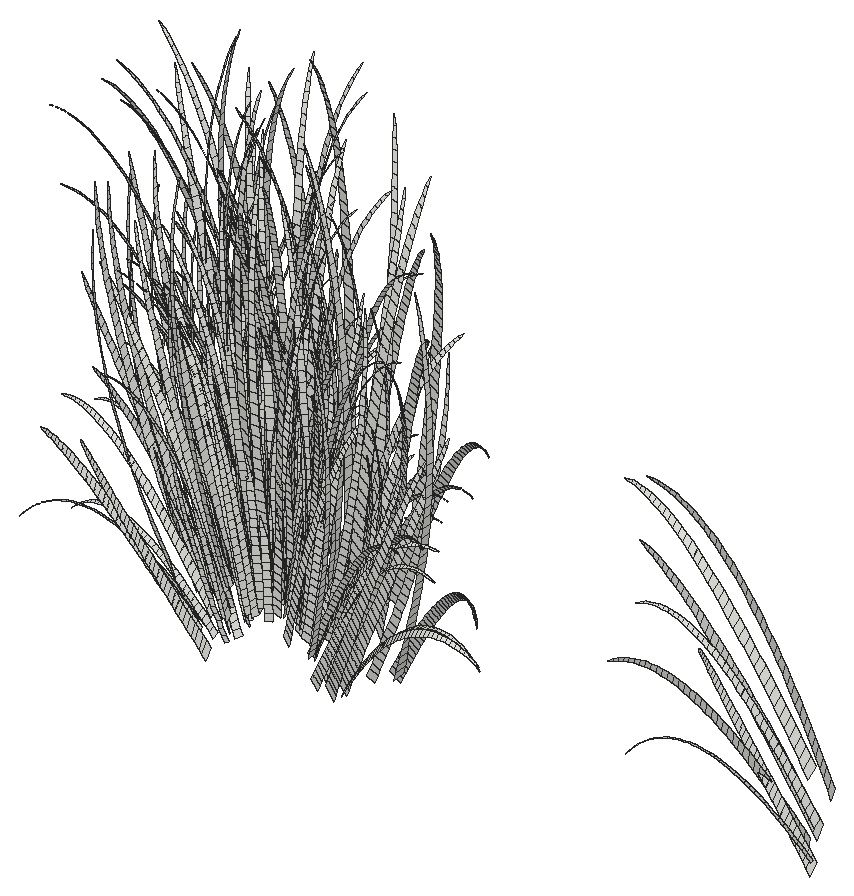
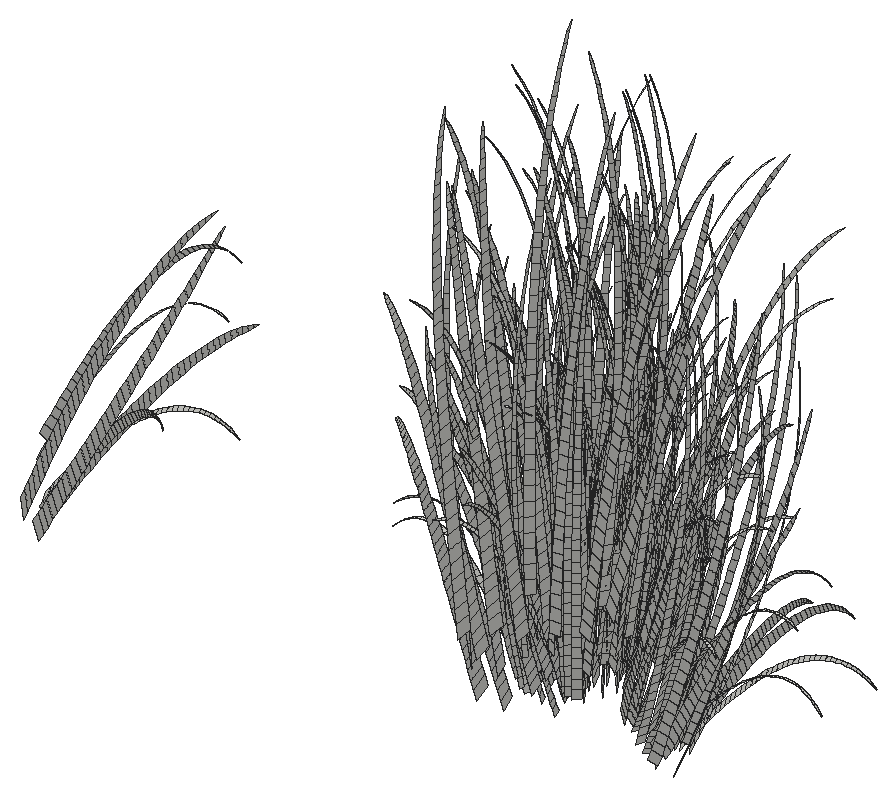
# SketchUp Ruby script. Lengths in inches.
U = 1.inch
M = Sketchup.active_model
def pt(a) = Geom::Point3d.new(a.map { |v| v * U })
def face(e, loops, mat)
  f = e.add_face(loops[0].map { |a| pt(a) })
  loops[1..].each { |l| e.add_face(l.map { |a| pt(a) }).erase! }
  f.material = f.back_material = mat if mat
  f
end
# faces: each face lists its corners as indices into pts; further lists are holes
def faces(e, pts, list, mat = nil) = list.each { |f| face(e, (f[0].is_a?(Array) ? f : [f]).map { |l| l.map { |i| pts[i] } }, mat) }
# xy, xz, yz: faces in a plane at the given z, y or x. An outline is a flat list of corners, or four numbers for a rectangle; further outlines are holes
def ring(l) = l.size == 4 ? [[l[0], l[1]], [l[2], l[1]], [l[2], l[3]], [l[0], l[3]]] : l.each_slice(2).to_a
def flat(e, list, mat, &to3) = list.each { |f| face(e, (f[0].is_a?(Array) ? f : [f]).map { |l| ring(l).map { |u, v| to3.(u, v) } }, mat) }
def xy(e, z, list, mat = nil) = flat(e, list, mat) { |x, y| [x, y, z] }
def xz(e, y, list, mat = nil) = flat(e, list, mat) { |x, z| [x, y, z] }
def yz(e, x, list, mat = nil) = flat(e, list, mat) { |y, z| [x, y, z] }
def lines(e, pts, list) = list.each { |a, b| e.add_line(pt(pts[a]), pt(pts[b])) }
# prism: a flat outline (further loops are holes) pulled along v
def prism(e, loops, v, mat = nil)
  f = face(e, loops, mat); d = Geom::Vector3d.new(v.map { |x| x * U })
  f.pushpull(f.normal.samedirection?(d) ? d.length : -d.length)
end
def box(e, o, s, mat = nil) = prism(e, [[o, [o[0] + s[0], o[1], o[2]], [o[0] + s[0], o[1] + s[1], o[2]], [o[0], o[1] + s[1], o[2]]]], [0, 0, s[2]], mat)
def at(x, y, z, deg = 0) = Geom::Transformation.translation(pt([x, y, z])) * Geom::Transformation.rotation(ORIGIN, Z_AXIS, deg.degrees)
def axes(o, x, y, z) = Geom::Transformation.new([*x, 0, *y, 0, *z, 0, *pt(o).to_a, 1])
def part(name) = M.definitions.add(name)
# library, detail: a bought-in or finely detailed component or shape, given as its bounding box
def library(name, o, s) = part(name).tap { |d| box(d.entities, o, s) }
def detail(e, o, s) = box(e.add_group.entities, o, s)
def put(e, d, t, mat = nil) = e.add_instance(d, t).tap { |i| i.material = mat if mat }
def group(e, t, mat = nil) = e.add_group.tap { |g| g.transformation = t; g.material = mat if mat }.entities
root = M.entities
c1 = part("fur_instance\#8")
p = [[-0.25,1.49,0.03],[0.25,-1.49,-0.03],[0.44,-1.47,1.51],[-0.05,1.47,1.57],[0.65,-1.44,3.05],[0.16,1.45,3.11],
  [0.86,-1.42,4.59],[0.38,1.44,4.65],[1.1,-1.39,6.13],[0.62,1.43,6.18],[1.34,-1.35,7.66],[0.875,1.42,7.72],
  [1.6,-1.32,9.19],[1.14,1.41,9.25],[1.88,-1.28,10.72],[1.43,1.41,10.78],[2.18,-1.24,12.25],[1.73,1.41,12.3],
  [2.49,-1.19,13.77],[2.05,1.41,13.82],[2.83,-1.15,15.29],[2.4,1.41,15.34],[3.18,-1.09,16.8],[2.76,1.42,16.85],
  [3.56,-1.03,18.31],[3.14,1.43,18.35],[3.96,-0.97,19.81],[3.55,1.44,19.85],[4.38,-0.91,21.3],[3.99,1.46,21.35],
  [4.84,-0.83,22.78],[4.45,1.48,22.83],[5.32,-0.76,24.26],[4.93,1.51,24.31],[5.82,-0.67,25.73],[5.45,1.54,25.77],
  [6.36,-0.59,27.18],[6,1.57,27.23],[6.93,-0.49,28.625],[6.58,1.61,28.67],[7.54,-0.39,30.05],[7.19,1.66,30.1],
  [8.18,-0.28,31.47],[7.84,1.71,31.51],[8.85,-0.16,32.86],[8.53,1.77,32.9],[9.57,-0.04,34.24],[9.25,1.83,34.27],
  [10.32,0.09,35.59],[10.02,1.9,35.625],[11.12,0.23,36.92],[10.82,1.97,36.95],[11.95,0.38,38.22],[11.67,2.06,38.25],
  [12.84,0.54,39.49],[12.57,2.14,39.52],[13.76,0.71,40.73],[13.51,2.24,40.76],[14.73,0.89,41.93],[14.49,2.34,41.95],
  [15.75,1.08,43.09],[15.52,2.45,43.11],[16.82,1.28,44.2],[16.6,2.5625,44.23],[17.93,1.5,45.27],[17.73,2.68,45.29],
  [19.08,1.73,46.28],[18.9,2.81,46.3],[20.29,1.97,47.24],[20.125,2.93,47.26],[21.53,2.22,48.13],[21.39,3.0625,48.15],
  [22.82,2.5,48.96],[22.7,3.1875,48.98],[24.14,2.8125,49.72],[24.06,3.3,49.73],[25.48,3.27,50.41]]
faces(c1.entities,p,[[0,1,2,3],[3,2,4,5],[5,4,6,7],[7,6,8,9],[9,8,10,11],[11,10,12,13],[13,12,14,15],[15,14,16,17],
  [17,16,18,19],[19,18,20,21],[21,20,22,23],[23,22,24,25],[25,24,26,27],[27,26,28,29],[29,28,30,31],[31,30,32,33],
  [33,32,34,35],[35,34,36,37],[37,36,38,39],[39,38,40,41],[41,40,42,43],[43,42,44,45],[45,44,46,47],[47,46,48,49],
  [49,48,50,51],[51,50,52,53],[53,52,54,55],[55,54,56,57],[57,56,58,59],[59,58,60,61],[61,60,62,63],[63,62,64,65],
  [65,64,66,67],[67,66,68,69],[69,68,70,71],[71,70,72,73],[73,72,74,75],[75,74,76]])
put(root,c1,axes([160.64,67.0625,2.47],[-0.11039,-0.00414,-0.3495],[0.07669,-0.1786,0.00651],[-0.14786,-0.06719,0.2791]))
put(root,c1,axes([161.22,65.8125,2.49],[-0.13594,0.15084,-0.11164],[-0.0609,-0.07291,-0.33491],[-0.13519,-0.09407,0.27953]))
put(root,c1,axes([158.93,69.58,2.69],[0.13391,-0.00422,0.37894],[-0.02725,0.21287,-0.08205],[-0.17659,-0.01268,0.31548]))
put(root,c1,axes([161.61,66.53,3.77],[-0.14992,0.10635,-0.20855],[-0.03569,-0.13875,-0.18978],[-0.12006,-0.06524,0.33426]))
put(root,c1,axes([161.6,67.96,3.64],[-0.13947,0.07457,-0.26376],[-0.03048,-0.16347,-0.05841],[-0.12421,-0.01975,0.3263]))
put(root,c1,axes([161.64,66.7,2.23],[-0.11214,0.07357,-0.29467],[-0.00419,-0.1506,-0.10442],[-0.13991,-0.03543,0.25192]))
put(root,c1,axes([160.7,70.26,10.22],[-0.16722,-0.14584,-0.14657],[0.18274,-0.19209,0.09427],[-0.0816,-0.06233,0.55718]))
put(root,c1,axes([159.23,71.21,3.75],[0.10956,-0.18152,0.25882],[0.13509,0.11782,0.19082],[-0.14519,0.00192,0.39222]))
put(root,c1,axes([160.22,69.17,3.12],[0.07012,-0.18381,0.20265],[0.10518,0.07075,0.29594],[-0.16336,-0.01173,0.29184]))
put(root,c1,axes([160.11,66.95,2.47],[0.11177,0.01694,0.37048],[-0.08915,0.18926,-0.03147],[-0.15727,-0.07147,0.29687]))
put(root,c1,axes([160.63,67.58,2.98],[0.07273,0.09595,0.27862],[-0.10249,0.16133,-0.212],[-0.15668,-0.03967,0.28211]))
put(root,c1,axes([159.15,68.47,3.74],[0.16226,-0.13696,0.26442],[0.06401,0.16282,0.19515],[-0.14822,-0.05035,0.39313]))
put(root,c1,axes([161.99,68.57,8.76],[-0.19486,-0.07064,-0.15993],[0.11436,-0.20339,0.01183],[-0.07048,-0.06892,0.50496]))
put(root,c1,axes([162.2,65.35,1.82],[-0.09839,0.14314,-0.01192],[-0.08354,-0.02419,-0.30566],[-0.11714,-0.08151,0.24221]))
put(root,c1,axes([161.59,68.2,2.32],[-0.01321,-0.17005,0.06481],[0.1141,-0.02557,0.30569],[-0.13946,0.01456,0.25678]))
put(root,c1,axes([162.7,69.16,6.58],[-0.18243,0.01895,-0.19563],[-0.00133,-0.1948,0.08688],[-0.09334,0.00298,0.40574]))
put(root,c1,axes([162.57,67.88,4.63],[-0.16023,0.03354,-0.19126],[-0.00898,-0.17162,0.02853],[-0.08895,-0.01176,0.36236]))
put(root,c1,axes([162.53,66.625,5.96],[-0.1494,0.14445,-0.05993],[-0.10862,-0.10225,-0.21391],[-0.08642,-0.08137,0.39881]))
put(root,c1,axes([160.01,68.125,4.63],[0.16036,-0.12824,0.26431],[0.05712,0.1633,0.18167],[-0.14465,-0.04914,0.38366]))
put(root,c1,axes([160.43,68.18,3.85],[0.12489,0.06673,0.27563],[-0.09958,0.18305,-0.12082],[-0.13573,-0.04611,0.36]))
put(root,c1,axes([162.82,66.73,4.46],[-0.15052,-0.00251,-0.18515],[0.03159,-0.16716,0.03488],[-0.08794,-0.02622,0.34898]))
put(root,c1,axes([162.91,68.06,3.03],[-0.10384,0.1021,-0.23208],[-0.0841,-0.12138,-0.04288],[-0.10059,0.0191,0.29067]))
put(root,c1,axes([162.55,68.69,5.18],[-0.10618,-0.13262,-0.04878],[0.13367,-0.1263,0.19427],[-0.08735,0.00279,0.37967]))
put(root,c1,axes([161.4,68.18,1.81],[0.10833,0.05099,0.24664],[-0.03776,0.16401,-0.19126],[-0.1393,0.01454,0.25647]))
put(root,c1,axes([162.52,70.78,11.4],[-0.09372,-0.20637,-0.07363],[0.22677,-0.12712,0.15354],[-0.08199,-0.04812,0.55353]))
put(root,c1,axes([160.94,69.19,4.28],[0.15491,-0.05585,0.29054],[0.02871,0.18789,-0.02061],[-0.13151,0.00174,0.35528]))
put(root,c1,axes([163.55,67.92,5.72],[-0.13836,0.10656,-0.19014],[-0.08729,-0.13946,-0.02631],[-0.08371,0.00267,0.36384]))
put(root,c1,axes([162.43,66.87,3.52],[0.03066,0.14936,0.05869],[-0.12804,0.07175,-0.24213],[-0.11455,-0.01821,0.30092]))
put(root,c1,axes([162.8,66.9375,7.41],[-0.03053,0.18634,0.11663],[-0.19498,0.03215,-0.20672],[-0.09234,-0.08694,0.42611]))
put(root,c1,axes([163.05,66.09,6],[-0.076,0.1669,0.09562],[-0.17144,-0.01335,-0.19918],[-0.07397,-0.09509,0.39348]))
put(root,c1,axes([163.36,67.9,6.33],[-0.14595,-0.08896,-0.08701],[0.11069,-0.159,0.08949],[-0.05969,-0.02587,0.41282]))
put(root,c1,axes([163.37,66.87,6.51],[-0.13003,0.1505,-0.04051],[-0.13515,-0.09639,-0.12681],[-0.0585,-0.05721,0.41915]))
put(root,c1,axes([163.36,69.73,10.31],[-0.20007,-0.1011,-0.05198],[0.13259,-0.20105,0.02025],[-0.03025,-0.05245,0.53866]))
put(root,c1,axes([163.86,69.61,11.42],[-0.23914,-0.05106,-0.06078],[0.08551,-0.22855,-0.0252],[-0.02809,-0.06875,0.5682]))
put(root,c1,axes([162.3,67.93,1.8125],[0.06974,-0.11239,0.27242],[0.09117,0.10684,0.0892],[-0.12045,0.03482,0.23783]))
put(root,c1,axes([161.48,69.49,3.4],[0.12819,-0.10555,0.27193],[0.08655,0.15023,0.02614],[-0.11644,0.02211,0.33646]))
put(root,c1,axes([162.47,66.64,2.11],[0.09888,-0.02928,0.28041],[-0.00291,0.15131,-0.01175],[-0.12783,-0.00918,0.22836]))
put(root,c1,axes([162.99,68.41,3.74],[-0.01787,-0.16163,0.13786],[0.14541,-0.01364,0.20157],[-0.09392,0.03632,0.30351]))
put(root,c1,axes([163.91,66.9,5.53],[-0.15295,0.08658,-0.10984],[-0.06653,-0.14152,-0.02919],[-0.05435,-0.02356,0.3759]))
put(root,c1,axes([163.57,68.36,3.76],[-0.08732,-0.12975,0.07004],[0.12156,-0.08169,0.22443],[-0.07712,0.04857,0.29461]))
put(root,c1,axes([164.39,69.47,11.48],[-0.24023,0.10194,-0.01182],[-0.08393,-0.20819,-0.06775],[-0.02132,-0.07588,0.56748]))
put(root,c1,axes([162.11,66.95,3.46],[0.13512,-0.04534,0.25565],[0.00767,0.16418,0.01521],[-0.11775,-0.01872,0.30933]))
put(root,c1,axes([164.27,66.88,5.49],[-0.16155,0.04363,-0.11105],[-0.02173,-0.15615,0.00187],[-0.05311,-0.02302,0.36735]))
put(root,c1,axes([164.18,68.14,5.39],[-0.13763,-0.08778,-0.02445],[0.09224,-0.14199,0.18002],[-0.06167,0.02548,0.35158]))
put(root,c1,axes([163.87,67.91,9.83],[-0.11071,0.19643,0.08485],[-0.20741,-0.05916,-0.14436],[-0.04649,-0.10158,0.50968]))
put(root,c1,axes([162.19,67.375,5.75],[0.12398,0.09622,0.18511],[-0.12468,0.16008,-0.11198],[-0.09878,-0.04719,0.39625]))
put(root,c1,axes([164.5,67.29,6.31],[-0.15275,-0.06369,-0.07605],[0.08272,-0.1606,0.08732],[-0.05298,-0.01559,0.38969]))
put(root,c1,axes([164.34,66.44,5.47],[-0.12167,0.12231,-0.08026],[-0.10576,-0.10199,-0.07795],[-0.05387,-0.03162,0.36369]))
put(root,c1,axes([162.84,67.73,5.89],[0.1073,0.11537,0.13468],[-0.12896,0.14123,-0.15523],[-0.09593,-0.0286,0.38067]))
put(root,c1,axes([164.74,66.98,5.32],[-0.15222,0.06371,-0.10078],[-0.04912,-0.14483,0.02613],[-0.04368,-0.00705,0.35627]))
put(root,c1,axes([164.89,66.57,7.14],[-0.18454,0.07316,-0.01839],[-0.05778,-0.16138,-0.04792],[-0.01906,-0.05522,0.43193]))
put(root,c1,axes([163.59,71.5625,10.07],[-0.03022,-0.22611,0.09029],[0.23429,-0.05028,0.11994],[-0.05481,-0.00145,0.5217]))
put(root,c1,axes([163.08,65.9,6.21],[0.08886,0.11953,0.22309],[-0.17307,0.12603,-0.0526],[-0.07674,-0.09865,0.40821]))
put(root,c1,axes([165,69.69,10.62],[-0.19122,-0.11806,-0.01455],[0.14538,-0.19433,0.04316],[-0.02276,-0.03764,0.53822]))
put(root,c1,axes([164,68.76,6.79],[-0.07059,-0.16734,0.04684],[0.17777,-0.08469,0.11217],[-0.04438,-0.00118,0.42241]))
put(root,c1,axes([165.09,67.4,6.18],[-0.1632,-0.04584,-0.02491],[0.06111,-0.16287,0.10545],[-0.03205,0.00396,0.38155]))
put(root,c1,axes([164.32,67.78,5.81],[-0.07809,-0.14325,0.0107],[0.15359,-0.09235,0.11164],[-0.04706,-0.00759,0.38378]))
put(root,c1,axes([165.17,68.24,7.07],[-0.18597,0.0618,-0.02273],[-0.04748,-0.17087,0.02426],[-0.01189,-0.02692,0.4292]))
put(root,c1,axes([163.43,67.35,3.28],[0.12505,0.02128,0.17693],[-0.02026,0.14885,-0.13694],[-0.09536,0.01811,0.27556]))
put(root,c1,axes([161.55,70.37,10.29],[0.23978,-0.07082,0.15768],[0.03022,0.22441,0.06362],[-0.07961,-0.06081,0.54364]))
put(root,c1,axes([164.3,68.31,8.43],[-0.04674,0.1979,-0.00041],[-0.20698,-0.02041,-0.04932],[-0.02674,-0.04637,0.47621]))
put(root,c1,axes([161.95,68.09,9.79],[0.21026,0.07749,0.17035],[-0.13208,0.20951,0.0486],[-0.06062,-0.09852,0.54406]))
put(root,c1,axes([162.31,69.1,7.84],[0.19711,0.03834,0.13931],[-0.07116,0.20343,-0.04176],[-0.07003,-0.0411,0.47276]))
put(root,c1,axes([163.66,67.91,4.64],[0.08378,-0.14307,0.16626],[0.13275,0.07958,0.06416],[-0.07048,0.0146,0.34149]))
put(root,c1,axes([165.46,65.47,5.33],[-0.14611,0.07417,-0.01085],[-0.0636,-0.12579,-0.04088],[-0.01571,-0.04551,0.35595]))
put(root,c1,axes([164.97,65.52,5.27],[-0.03907,0.14419,0.04289],[-0.15068,-0.00691,-0.10234],[-0.04404,-0.05511,0.34471]))
put(root,c1,axes([165.77,66.39,7.37],[-0.18895,0.06999,0.02245],[-0.05996,-0.16418,-0.04942],[-0.00199,-0.06326,0.44045]))
put(root,c1,axes([164.81,68.33,9.8125],[-0.07149,0.20688,0.05021],[-0.22153,-0.04139,-0.03916],[-0.01557,-0.07173,0.51835]))
put(root,c1,axes([165.41,67.78,4.4],[-0.12985,-0.07677,0.07158],[0.09092,-0.12597,0.14453],[-0.01646,0.03757,0.31821]))
put(root,c1,axes([164.9,66.36,5.48],[0.0007,0.15498,-0.03624],[-0.15701,0.01919,-0.0982],[-0.04789,-0.01409,0.35225]))
put(root,c1,axes([162.6875,69.85,8.71],[0.21533,-0.00022,0.14201],[-0.02985,0.21622,-0.04212],[-0.07083,-0.0307,0.48991]))
put(root,c1,axes([164.8125,69.9,6.69],[-0.05762,-0.17661,0.09378],[0.18885,-0.07013,0.07584],[-0.02585,0.00825,0.42914]))
put(root,c1,axes([165.52,66.12,6.67],[-0.11204,0.14362,0.03398],[-0.14775,-0.08605,-0.03808],[-0.00899,-0.05843,0.41243]))
put(root,c1,axes([164.47,66.88,5.72],[0.07256,0.13813,0.01061],[-0.14853,0.08916,-0.10968],[-0.05042,-0.01484,0.37084]))
put(root,c1,axes([166.33,68.28,7.88],[-0.20122,0.04978,0.02765],[-0.03696,-0.18587,0.02525],[0.00919,-0.0352,0.4569]))
put(root,c1,axes([165.13,69.16,7.99],[-0.07053,-0.17965,0.10788],[0.19435,-0.08267,0.06265],[-0.01549,0.01046,0.44704]))
put(root,c1,axes([165.74,67,5.46],[-0.12044,0.11617,-0.06507],[-0.11184,-0.10532,0.07409],[-0.00291,0.00808,0.35453]))
put(root,c1,axes([164.14,66.82,6.85],[0.1306,0.09776,0.12408],[-0.13059,0.14634,-0.04229],[-0.05761,-0.05634,0.41276]))
put(root,c1,axes([166,67,5.7],[-0.14146,0.09732,-0.03277],[-0.08974,-0.12702,0.09515],[0.00654,0.00629,0.36155]))
put(root,c1,axes([165.3125,66.14,7.21],[-0.02865,0.1632,0.13083],[-0.19416,0.00105,-0.04665],[-0.01776,-0.09378,0.4187]))
put(root,c1,axes([163.26,68.21,9.33],[0.21896,0.00722,0.14738],[-0.05367,0.20894,0.06409],[-0.06377,-0.07981,0.49923]))
put(root,c1,axes([165.19,66.79,5.79],[-0.005,0.15882,-0.01867],[-0.16818,0.01184,-0.02587],[-0.01594,-0.02637,0.37698]))
put(root,c1,axes([166.17,68.37,4.09],[-0.15178,-0.03817,0.09021],[0.05761,-0.14672,0.13772],[0.01323,0.03497,0.32535]))
put(root,c1,axes([166.14,68.04,4.65],[-0.14817,-0.05096,0.10268],[0.07099,-0.14472,0.13123],[0.01339,0.03539,0.32926]))
put(root,c1,axes([165.7,65.7,5.82],[-0.04364,0.1509,0.04181],[-0.16335,-0.02313,-0.02043],[-0.0082,-0.05328,0.37608]))
put(root,c1,axes([164.3,66.81,6.55],[0.16328,0.03799,0.12354],[-0.06943,0.16853,-0.0179],[-0.05845,-0.04464,0.39911]))
put(root,c1,axes([165.89,68.17,5.49],[-0.0829,-0.13844,0.09301],[0.15279,-0.09132,0.04718],[-0.00308,0.00854,0.37496]))
put(root,c1,axes([164.4375,68.7,6.83],[0.11915,-0.15444,0.11959],[0.14734,0.10329,0.01409],[-0.04397,-0.00116,0.41847]))
put(root,c1,axes([163.91,68.36,6.46],[0.18469,-0.02182,0.1026],[0.00322,0.18141,-0.06268],[-0.05045,-0.00814,0.41143]))
put(root,c1,axes([166.02,67.02,8.61],[-0.06667,0.19226,0.05915],[-0.20819,-0.04319,-0.00198],[0.00188,-0.06909,0.48578]))
put(root,c1,axes([166.14,68.83,6.34],[-0.10911,-0.1372,0.1051],[0.15387,-0.1168,0.04236],[0.00736,0.00708,0.40712]))
put(root,c1,axes([164.76,70.77,5.5],[0.05449,-0.17808,0.19773],[0.18828,0.03949,-0.026],[-0.02035,0.04645,0.39347]))
put(root,c1,axes([164.5625,66.2,5.34],[0.15146,0.01629,0.10652],[-0.04117,0.15418,-0.02273],[-0.05245,-0.03078,0.35407]))
put(root,c1,axes([165.28,69.19,6.84],[0.00836,-0.18662,0.11674],[0.19508,-0.00753,0.01588],[-0.01463,0.00988,0.4222]))
put(root,c1,axes([164.25,68.6,8.21],[0.12224,-0.1724,0.03147],[0.17004,0.09672,0.03094],[-0.02457,-0.03858,0.46994]))
put(root,c1,axes([165.47,71.77,9.61],[-0.01914,-0.22341,0.14227],[0.23668,-0.03758,0.00754],[-0.0042,0.01167,0.5122]))
put(root,c1,axes([166.42,65.51,5.34],[-0.08483,0.12977,0.03637],[-0.13576,-0.06868,0.01436],[0.01015,-0.0438,0.35695]))
put(root,c1,axes([164.67,66.92,7.01],[0.13112,0.1119,0.04642],[-0.13781,0.13647,-0.01148],[-0.02271,-0.04835,0.42618]))
put(root,c1,axes([163.78,67.25,9.36],[0.22597,0.02863,0.10796],[-0.07525,0.20019,0.13019],[-0.03474,-0.10937,0.51158]))
put(root,c1,axes([166.63,70.6,7.58],[-0.12335,-0.15584,0.12717],[0.17408,-0.13265,0.02266],[0.01997,0.00343,0.46197]))
put(root,c1,axes([165.9,68.51,7.9375],[-0.03248,-0.18789,0.03246],[0.20264,-0.04691,-0.01246],[0.00277,-0.0305,0.45814]))
put(root,c1,axes([165.3,70.71,5.47],[0.06236,-0.17527,0.19539],[0.18475,0.04701,-0.03446],[-0.02024,0.04621,0.39144]))
put(root,c1,axes([163.42,70.18,11.4],[0.24246,-0.09581,0.04741],[0.07374,0.21618,0.03906],[-0.03158,-0.05994,0.56838]))
put(root,c1,axes([165.65,69.22,8.11],[0.00458,-0.19714,0.03462],[0.20895,-0.01368,-0.00104],[-0.00501,-0.02872,0.46671]))
put(root,c1,axes([165.11,66.2,8.97],[0.08928,0.17665,0.16183],[-0.22737,0.09539,0.05927],[-0.00818,-0.11915,0.51927]))
put(root,c1,axes([164.59,68.33,5.63],[0.167,0.03821,0.03014],[-0.05354,0.16593,-0.1048],[-0.03226,0.00399,0.38398]))
put(root,c1,axes([166.9,67.23,4.97],[-0.11227,0.12169,-0.01571],[-0.11695,-0.0983,0.09825],[0.0234,-0.00238,0.35291]))
put(root,c1,axes([166.37,68.5,10.47],[-0.01737,0.2214,0.05487],[-0.24332,0.00145,0.03189],[0.01003,-0.07326,0.54284]))
put(root,c1,axes([166.125,65.79,7.44],[-0.01068,0.1751,0.14296],[-0.21108,0.00073,0.04004],[0.01667,-0.10172,0.45077]))
put(root,c1,axes([166.6,68.3,8.15],[-0.03706,0.19452,0.0025],[-0.2058,-0.02021,0.04233],[0.01369,-0.04269,0.4672]))
put(root,c1,axes([166.13,67.62,8.14],[0.00321,0.19067,0.02092],[-0.20749,0.01649,0.04397],[0.01444,-0.0534,0.46311]))
put(root,c1,axes([165.97,66.97,6.03],[0.0444,0.15353,-0.02873],[-0.16709,0.05572,0.00025],[-0.00083,-0.02443,0.38596]))
put(root,c1,axes([164.59,67.77,7.43],[0.19137,0.02245,0.03812],[-0.04546,0.1843,-0.01629],[-0.02307,-0.03624,0.44138]))
put(root,c1,axes([165.62,69.2,9.32],[0.0752,-0.20516,0.02464],[0.21175,0.0536,-0.02901],[0.00304,-0.03339,0.50163]))
put(root,c1,axes([165.44,70.36,5.36],[0.1059,-0.15637,0.15831],[0.16025,0.08485,-0.11228],[-0.00207,0.04487,0.3837]))
put(root,c1,axes([167.84,69.14,9.93],[-0.20879,-0.09834,0.1321],[0.10662,-0.20129,-0.08744],[0.06463,-0.06137,0.52082]))
put(root,c1,axes([166.16,67.43,5.97],[0.04623,0.15623,-0.10375],[-0.16763,0.05842,0.01792],[0.01628,0.0028,0.37652]))
put(root,c1,axes([165.44,66.62,5.85],[0.15712,0.04243,0.01115],[-0.06087,0.1538,-0.0283],[-0.01337,-0.02475,0.37716]))
put(root,c1,axes([166.64,67.09,5.42],[-0.02615,-0.15514,0.08978],[0.1636,-0.03862,-0.04775],[0.02391,-0.00243,0.36067]))
put(root,c1,axes([165.34,68.37,5.37],[0.17226,-0.02677,0.04434],[0.01787,0.15893,-0.17055],[-0.01798,0.04104,0.34767]))
put(root,c1,axes([165.24,69.57,7.86],[0.17834,-0.11625,0.08266],[0.1071,0.16149,-0.09447],[-0.01558,0.01053,0.44981]))
put(root,c1,axes([168.01,67.0625,7],[-0.15292,0.11854,0.12624],[-0.12574,-0.14279,0.04956],[0.05301,-0.06232,0.4383]))
put(root,c1,axes([167.25,68.91,4.93],[-0.09023,-0.13424,0.18354],[0.14991,-0.10591,-0.00994],[0.04513,0.02354,0.36032]))
put(root,c1,axes([166.81,66.69,5.33],[0.01188,0.15545,-0.07184],[-0.16156,0.0237,0.07132],[0.03067,-0.00873,0.35494]))
put(root,c1,axes([166.75,65.76,5.75],[-0.00201,0.1516,0.05729],[-0.16575,-0.0022,0.09935],[0.04109,-0.06021,0.3647]))
put(root,c1,axes([168.14,67.33,4.33],[-0.15312,0.05179,0.12153],[-0.03636,-0.15379,0.12597],[0.06399,-0.0008,0.33763]))
put(root,c1,axes([166.16,66.54,5.63],[0.13491,0.07893,-0.02845],[-0.09527,0.13412,-0.00523],[0.005,-0.02625,0.36875]))
put(root,c1,axes([166.88,69.04,4.84],[0.00974,-0.16765,0.16266],[0.17627,-0.01134,-0.08044],[0.03031,0.03221,0.35757]))
put(root,c1,axes([167.72,66.65,5.01],[-0.12808,-0.08127,0.17105],[0.08472,-0.13879,-0.03962],[0.07069,-0.01437,0.33524]))
put(root,c1,axes([166.82,72.16,11.75],[-0.01557,-0.2472,0.11257],[0.25666,-0.03446,-0.11464],[0.04868,-0.01385,0.56337]))
put(root,c1,axes([166.05,68.8,11.2],[0.1638,0.16225,0.02835],[-0.19372,0.16204,0.06129],[0.00656,-0.07857,0.56406]))
put(root,c1,axes([166.55,67.81,4.25],[0.06075,-0.14439,0.11282],[0.14535,0.04045,-0.11615],[0.02704,0.02874,0.31908]))
put(root,c1,axes([166.96,67.84,9.05],[0.00546,0.20018,0.07075],[-0.21886,0.00452,0.13393],[0.05427,-0.07952,0.48166]))
put(root,c1,axes([166.01,69.05,8.9],[0.1489,-0.1631,0.00196],[0.16131,0.12724,-0.0384],[0.00665,-0.0349,0.49014]))
put(root,c1,axes([168.57,68.03,5.81],[-0.17727,-0.00884,0.19718],[0.01815,-0.18643,0.05134],[0.08203,-0.01667,0.38902]))
put(root,c1,axes([165.52,68.81,10.45],[0.24085,-0.01288,-0.01594],[-0.00713,0.21681,0.06326],[0.00207,-0.07616,0.53545]))
put(root,c1,axes([168.66,68.4,7.44],[-0.19467,0.01004,0.22404],[-0.00781,-0.20399,0.04036],[0.09618,-0.03688,0.42982]))
put(root,c1,axes([165.53,69.48,11.5625],[0.24462,0.04853,-0.00958],[-0.07419,0.22591,0.06737],[0.00661,-0.07917,0.56836]))
put(root,c1,axes([166.29,67.41,5.75],[0.16085,-0.07091,-0.00868],[0.05991,0.14859,-0.10356],[0.01607,0.00276,0.37166]))
put(root,c1,axes([168.27,66.49,4.31],[-0.09933,0.11915,0.09682],[-0.11277,-0.10305,0.14649],[0.07419,-0.02845,0.33155]))
put(root,c1,axes([167.01,65.87,7.53],[0.1142,0.15271,0.07486],[-0.18421,0.10064,0.13224],[0.02836,-0.10071,0.46512]))
put(root,c1,axes([167.44,66.91,4.26],[0.01848,-0.15029,0.09797],[0.14831,0.00119,-0.12824],[0.05045,0.01072,0.31409]))
put(root,c1,axes([166.15,67.96,8.99],[0.21441,0.03504,-0.02755],[-0.05444,0.19871,0.04867],[0.01191,-0.06374,0.49276]))
put(root,c1,axes([166.66,66.59,5.26],[0.15483,0.02452,-0.08835],[-0.03742,0.15266,-0.04583],[0.03016,-0.00858,0.34899]))
put(root,c1,axes([167.15,66.39,4.93],[0.12172,0.08749,-0.09823],[-0.09805,0.12464,0.01693],[0.03543,-0.01566,0.34464]))
put(root,c1,axes([168.69,70.26,6.49],[-0.10531,-0.16415,0.20039],[0.16955,-0.12413,-0.09552],[0.08116,-0.00102,0.4282]))
put(root,c1,axes([166.7,67.3,6.65],[0.15584,0.0797,-0.11547],[-0.0923,0.15744,0.00315],[0.04105,-0.01815,0.39937]))
put(root,c1,axes([169.75,68.26,7.57],[-0.20296,0.04396,0.25147],[-0.06114,-0.20583,-0.00189],[0.10319,-0.08007,0.46398]))
put(root,c1,axes([168.47,66.9,5.41],[-0.05241,0.16147,0.07727],[-0.15892,-0.06034,0.18232],[0.08415,-0.0479,0.3696]))
put(root,c1,axes([167.43,66.85,5.91],[0.10935,0.12723,-0.0806],[-0.13524,0.11022,0.08276],[0.04716,-0.03593,0.38648]))
put(root,c1,axes([168.94,66.15,3.65],[-0.13363,0.01209,0.24348],[-0.02341,-0.15821,0.02454],[0.10585,-0.04288,0.29749]))
put(root,c1,axes([167.64,65.54,4.49],[0.04868,0.13833,-0.04452],[-0.13249,0.04478,0.16098],[0.07098,-0.0404,0.31175]))
put(root,c1,axes([167.1,68.62,3.92],[0.15705,-0.06817,-0.01855],[0.04537,0.13415,-0.23216],[0.04015,0.05663,0.29621]))
put(root,c1,axes([168.21,66.96,3.72],[-0.0035,0.15221,-0.13037],[-0.13811,0.0204,0.18439],[0.08356,0.01425,0.28222]))
put(root,c1,axes([167.16,68.01,9.67],[0.18476,0.1259,-0.03463],[-0.14125,0.16417,0.15823],[0.05053,-0.09421,0.50755]))
put(root,c1,axes([169.22,67.04,4.53],[-0.105,0.10997,0.20265],[-0.1047,-0.1341,0.17455],[0.11569,-0.04687,0.32514]))
put(root,c1,axes([167.42,68.72,6.91],[0.18917,-0.06704,-0.06686],[0.05451,0.17895,-0.10326],[0.03727,-0.0106,0.43133]))
put(root,c1,axes([168.76,67.5,1.76],[-0.02967,-0.12807,0.22483],[0.11753,-0.07372,-0.14887],[0.10049,0.02798,0.22698]))
put(root,c1,axes([167.01,69.07,8.93],[0.21551,0.00607,-0.13742],[-0.0172,0.21045,-0.03067],[0.05502,-0.03283,0.47913]))
put(root,c1,axes([167.5,67.71,6.93],[0.18544,-0.04972,-0.1199],[0.04511,0.1779,-0.04118],[0.05175,-0.03943,0.42412]))
put(root,c1,axes([170.33,69.2,8.01],[-0.13857,0.17143,0.18015],[-0.17196,-0.14956,0.18932],[0.11106,-0.06322,0.48777]))
put(root,c1,axes([169.66,69.35,3.87],[-0.08271,-0.14836,0.25336],[0.14839,-0.11682,-0.11362],[0.10275,0.01753,0.34702]))
put(root,c1,axes([167.95,67.73,3.55],[0.1392,0.01865,-0.19659],[-0.04604,0.15192,-0.11441],[0.07206,0.03039,0.28637]))
put(root,c1,axes([167.6,69.6875,8.92],[0.2045,-0.09371,-0.11076],[0.08595,0.19464,-0.09275],[0.05645,-0.03369,0.4916]))
put(root,c1,axes([168.07,71.22,8.32],[0.13505,-0.18869,0.02697],[0.17317,0.11473,-0.23558],[0.07413,0.01575,0.4615]))
put(root,c1,axes([170.15,68.18,6.88],[-0.05009,0.1972,0.12811],[-0.20341,-0.06615,0.21296],[0.10198,-0.07913,0.45854]))
put(root,c1,axes([169.74,67.67,4.17],[-0.05226,0.17384,0.04608],[-0.14605,-0.06174,0.27189],[0.11826,-0.02606,0.33853]))
put(root,c1,axes([169.3,65.9375,2.1],[-0.0259,0.13847,0.08839],[-0.10293,-0.05886,0.26708],[0.12297,-0.03787,0.2304]))
put(root,c1,axes([168.2,67.41,6.72],[0.19428,0.00099,-0.13011],[-0.00447,0.1857,0.01775],[0.05358,-0.05088,0.43173]))
put(root,c1,axes([169.53,67.67,2.35],[-0.0586,-0.13145,0.25194],[0.10919,-0.10295,-0.16429],[0.12358,0.00811,0.25105]))
put(root,c1,axes([168.44,66.77,3.32],[0.11365,-0.08796,-0.13302],[0.06535,0.12495,-0.18142],[0.09174,-0.00314,0.27875]))
put(root,c1,axes([168.96,68.98,3.85],[0.12182,-0.13641,-0.05722],[0.10481,0.11532,-0.25636],[0.0972,0.01658,0.32827]))
put(root,c1,axes([168.71,68.15,4.4375],[0.15112,-0.07348,-0.15621],[0.04279,0.15836,-0.20373],[0.095,0.01621,0.32084]))
put(root,c1,axes([170.41,67.97,7.79],[0.03711,0.21617,0.09276],[-0.22705,0.0107,0.25479],[0.10293,-0.10542,0.49477]))
put(root,c1,axes([169.7,68.18,6.04],[0.10459,0.17012,-0.10766],[-0.16118,0.10117,0.20027],[0.09662,-0.055,0.42437]))
put(root,c1,axes([171.23,68.55,1.99],[-0.11534,0.10838,0.24896],[-0.07338,-0.1624,0.25205],[0.15325,-0.01897,0.29298]))
put(root,c1,axes([169.22,66.17,3.82],[0.13705,0.06092,-0.24143],[-0.03897,0.15511,0.08813],[0.11117,-0.04504,0.31244]))
put(root,c1,axes([170.93,69.52,4.5625],[-0.04683,-0.20253,0.13494],[0.1704,-0.05617,-0.28372],[0.13472,-0.02969,0.38568]))
put(root,c1,axes([169.49,66.62,3.24],[0.14053,0.00256,-0.25431],[0.0115,0.16488,-0.00221],[0.11001,-0.04457,0.30917]))
put(root,c1,axes([169.72,67.55,3.5625],[0.11573,-0.11352,-0.17299],[0.09518,0.13737,-0.20258],[0.11423,-0.02517,0.32701]))
put(root,c1,axes([170.5625,65.75,2.08],[0.04443,0.16095,0.1082],[-0.13761,-0.02397,0.33152],[0.13789,-0.09974,0.2801]))
put(root,c1,axes([171.09,72.45,7.95],[0.03522,-0.24577,0.05534],[0.23308,0.0235,-0.26379],[0.10852,-0.02206,0.51462]))
put(root,c1,axes([170.89,66.45,2.2],[0.00679,0.17207,0.10989],[-0.13694,-0.04896,0.33579],[0.14998,-0.07528,0.28652]))
put(root,c1,axes([170.6,70.35,7.44],[0.1074,-0.20139,-0.09354],[0.19115,0.11076,-0.2385],[0.10824,-0.04151,0.48371]))
put(root,c1,axes([169.96,69.12,4.6],[0.15027,-0.10781,-0.18095],[0.0791,0.16599,-0.22838],[0.11882,-0.00407,0.36105]))
put(root,c1,axes([173.15,68.63,2.75],[-0.15284,0.01805,0.42901],[-0.06641,-0.2167,0.01891],[0.18229,-0.0915,0.34824]))
put(root,c1,axes([170.84,67.28,2.26],[0.12633,-0.01434,-0.33979],[0.03003,0.18353,-0.05493],[0.15045,-0.04633,0.28189]))
put(root,c1,axes([171.06,66.42,2.13],[0.13942,0.04831,-0.34302],[0.00816,0.17572,0.1089],[0.15278,-0.07668,0.29185]))
put(root,c1,axes([171.31,70.61,5.98],[0.12813,-0.17071,-0.17976],[0.14324,0.15198,-0.29056],[0.14651,-0.03228,0.41943]))
put(root,c1,axes([172.58,69.0625,2.38],[0.07286,-0.17069,-0.21842],[0.13329,0.1313,-0.33824],[0.176,-0.05419,0.32974]))
put(root,c1,axes([202.86,68.45,7.11],[-0.18691,0.1568,-0.23935],[-0.06787,-0.16218,-0.27405],[-0.15492,-0.08418,0.43132]))
put(root,c1,axes([202.09,71.27,4.24],[-0.09014,-0.18111,-0.08882],[0.15594,-0.13199,0.32093],[-0.15035,0.00199,0.40617]))
put(root,c1,axes([202.125,70.05,2.34],[0.01897,-0.21218,0.0586],[0.13531,-0.01729,0.38322],[-0.17657,-0.01268,0.31544]))
put(root,c1,axes([202.71,68.3125,2.6],[-0.03242,-0.16161,-0.19656],[0.13271,-0.12456,0.32589],[-0.17032,-0.04313,0.30667]))
put(root,c1,axes([204.09,67.32,4.85],[-0.17146,0.07712,-0.27655],[0.00216,-0.17859,-0.14821],[-0.13359,-0.07259,0.37194]))
put(root,c1,axes([203.74,67.44,1.72],[-0.07927,0.1771,-0.13212],[-0.09456,-0.05104,-0.31736],[-0.15384,-0.03896,0.27701]))
put(root,c1,axes([203.95,67.0625,2.47],[-0.11039,-0.00414,-0.3495],[0.07669,-0.1786,0.00651],[-0.14786,-0.06719,0.2791]))
